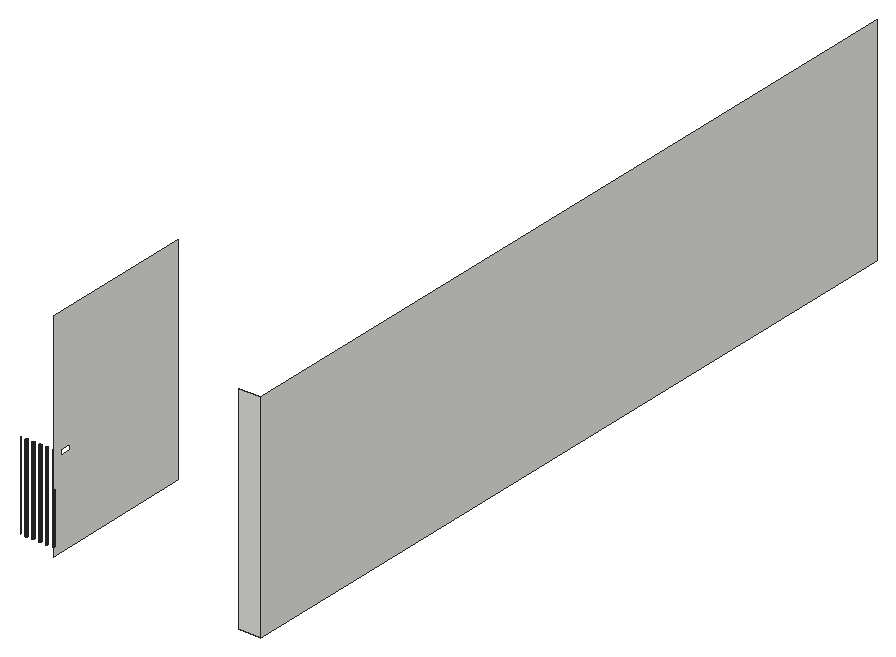
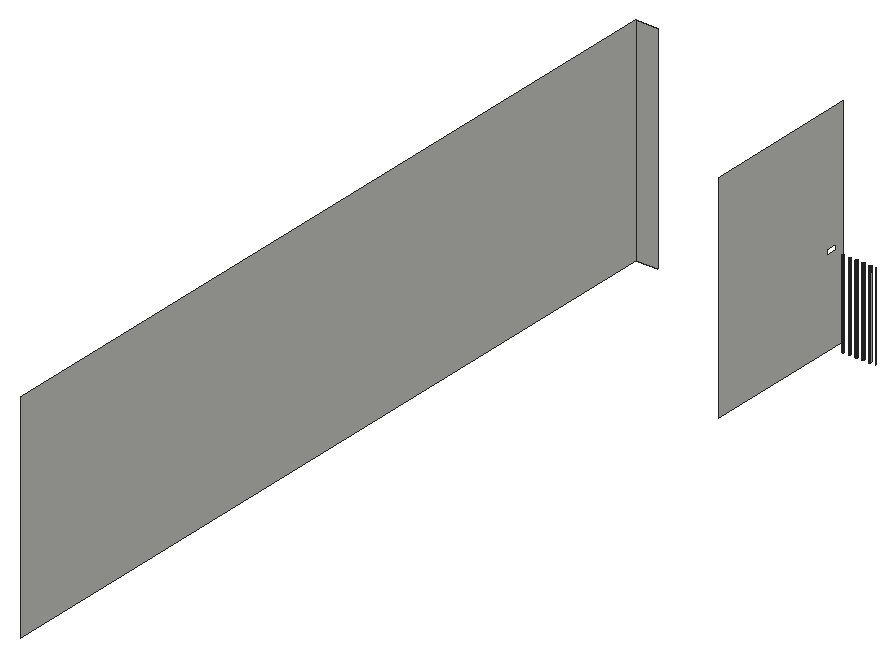
# SketchUp Ruby script. Lengths in inches.
U = 1.inch
M = Sketchup.active_model
def pt(a) = Geom::Point3d.new(a.map { |v| v * U })
def face(e, loops, mat)
  f = e.add_face(loops[0].map { |a| pt(a) })
  loops[1..].each { |l| e.add_face(l.map { |a| pt(a) }).erase! }
  f.material = f.back_material = mat if mat
  f
end
# faces: each face lists its corners as indices into pts; further lists are holes
def faces(e, pts, list, mat = nil) = list.each { |f| face(e, (f[0].is_a?(Array) ? f : [f]).map { |l| l.map { |i| pts[i] } }, mat) }
# xy, xz, yz: faces in a plane at the given z, y or x. An outline is a flat list of corners, or four numbers for a rectangle; further outlines are holes
def ring(l) = l.size == 4 ? [[l[0], l[1]], [l[2], l[1]], [l[2], l[3]], [l[0], l[3]]] : l.each_slice(2).to_a
def flat(e, list, mat, &to3) = list.each { |f| face(e, (f[0].is_a?(Array) ? f : [f]).map { |l| ring(l).map { |u, v| to3.(u, v) } }, mat) }
def xy(e, z, list, mat = nil) = flat(e, list, mat) { |x, y| [x, y, z] }
def xz(e, y, list, mat = nil) = flat(e, list, mat) { |x, z| [x, y, z] }
def yz(e, x, list, mat = nil) = flat(e, list, mat) { |y, z| [x, y, z] }
def lines(e, pts, list) = list.each { |a, b| e.add_line(pt(pts[a]), pt(pts[b])) }
# prism: a flat outline (further loops are holes) pulled along v
def prism(e, loops, v, mat = nil)
  f = face(e, loops, mat); d = Geom::Vector3d.new(v.map { |x| x * U })
  f.pushpull(f.normal.samedirection?(d) ? d.length : -d.length)
end
def box(e, o, s, mat = nil) = prism(e, [[o, [o[0] + s[0], o[1], o[2]], [o[0] + s[0], o[1] + s[1], o[2]], [o[0], o[1] + s[1], o[2]]]], [0, 0, s[2]], mat)
def at(x, y, z, deg = 0) = Geom::Transformation.translation(pt([x, y, z])) * Geom::Transformation.rotation(ORIGIN, Z_AXIS, deg.degrees)
def axes(o, x, y, z) = Geom::Transformation.new([*x, 0, *y, 0, *z, 0, *pt(o).to_a, 1])
def part(name) = M.definitions.add(name)
# library, detail: a bought-in or finely detailed component or shape, given as its bounding box
def library(name, o, s) = part(name).tap { |d| box(d.entities, o, s) }
def detail(e, o, s) = box(e.add_group.entities, o, s)
def put(e, d, t, mat = nil) = e.add_instance(d, t).tap { |i| i.material = mat if mat }
def group(e, t, mat = nil) = e.add_group.tap { |g| g.transformation = t; g.material = mat if mat }.entities
root = M.entities
xy(root,409.875,[[500.17,133.41,499.96,133.44,499.76,133.52,499.59,133.65,499.46,133.82,499.38,134.02,499.36,134.23,499.38,134.4375,499.46,134.63,499.59,134.8,499.76,134.93,499.96,135.01,500.17,135.04,500.38,135.01,500.57,134.93,500.74,134.8,500.87,134.63,500.95,134.4375,500.98,134.23,500.95,134.02,500.87,133.82,500.74,133.65,500.57,133.52,500.38,133.44],[505.42,133.41,505.21,133.44,505.01,133.52,504.84,133.65,504.71,133.82,504.63,134.02,504.61,134.23,504.63,134.4375,504.71,134.63,504.84,134.8,505.01,134.93,505.21,135.01,505.42,135.04,505.63,135.01,505.82,134.93,505.99,134.8,506.12,134.63,506.2,134.4375,506.23,134.23,506.2,134.02,506.12,133.82,505.99,133.65,505.82,133.52,505.63,133.44],[510.67,133.41,510.46,133.44,510.26,133.52,510.09,133.65,509.96,133.82,509.88,134.02,509.86,134.23,509.88,134.4375,509.96,134.63,510.09,134.8,510.26,134.93,510.46,135.01,510.67,135.04,510.88,135.01,511.07,134.93,511.24,134.8,511.37,134.63,511.45,134.4375,511.48,134.23,511.45,134.02,511.37,133.82,511.24,133.65,511.07,133.52,510.88,133.44],[515.92,133.41,515.71,133.44,515.51,133.52,515.34,133.65,515.21,133.82,515.13,134.02,515.11,134.23,515.13,134.4375,515.21,134.63,515.34,134.8,515.51,134.93,515.71,135.01,515.92,135.04,516.13,135.01,516.32,134.93,516.49,134.8,516.62,134.63,516.7,134.4375,516.73,134.23,516.7,134.02,516.62,133.82,516.49,133.65,516.32,133.52,516.13,133.44],[521.23,133.41,521.02,133.44,520.82,133.52,520.66,133.65,520.53,133.82,520.45,134.02,520.42,134.23,520.45,134.4375,520.53,134.63,520.66,134.8,520.82,134.93,521.02,135.01,521.23,135.04,521.44,135.01,521.64,134.93,521.8,134.8,521.93,134.63,522.02,134.4375,522.04,134.23,522.02,134.02,521.93,133.82,521.8,133.65,521.64,133.52,521.44,133.44]])
xz(root,124.5,[[673.48,409.875,690.4375,577.875]])
yz(root,528.75,[[[124.5,409.875,246,577.875],[131.37,477.08,140.67,481.27]]])
yz(root,690.4375,[[124.5,409.875,724.5,577.875]])
p = [[499.76,133.52,409.875],[499.96,133.44,409.875],[499.96,133.44,477.08],[499.76,133.52,477.08],[500.17,133.41,409.875],[500.17,133.41,477.08],
  [500.38,133.44,409.875],[500.38,133.44,477.08],[500.57,133.52,409.875],[500.57,133.52,477.08],[505.01,133.52,409.875],[505.21,133.44,409.875],
  [505.21,133.44,477.08],[505.01,133.52,477.08],[505.42,133.41,409.875],[505.42,133.41,477.08],[505.63,133.44,409.875],[505.63,133.44,477.08],
  [505.82,133.52,409.875],[505.82,133.52,477.08],[510.26,133.52,409.875],[510.46,133.44,409.875],[510.46,133.44,477.08],[510.26,133.52,477.08],
  [510.67,133.41,409.875],[510.67,133.41,477.08],[510.88,133.44,409.875],[510.88,133.44,477.08],[511.07,133.52,409.875],[511.07,133.52,477.08],
  [515.51,133.52,409.875],[515.71,133.44,409.875],[515.71,133.44,477.08],[515.51,133.52,477.08],[515.92,133.41,409.875],[515.92,133.41,477.08],
  [516.13,133.44,409.875],[516.13,133.44,477.08],[516.32,133.52,409.875],[516.32,133.52,477.08],[520.82,133.52,409.875],[521.02,133.44,409.875],
  [521.02,133.44,477.08],[520.82,133.52,477.08],[521.23,133.41,409.875],[521.23,133.41,477.08],[521.44,133.44,409.875],[521.44,133.44,477.08],
  [521.64,133.52,409.875],[521.64,133.52,477.08],[499.59,133.65,409.875],[499.59,133.65,477.08],[500.74,133.65,409.875],[500.74,133.65,477.08],
  [504.84,133.65,409.875],[504.84,133.65,477.08],[505.99,133.65,409.875],[505.99,133.65,477.08],[510.09,133.65,409.875],[510.09,133.65,477.08],
  [511.24,133.65,409.875],[511.24,133.65,477.08],[515.34,133.65,409.875],[515.34,133.65,477.08],[516.49,133.65,409.875],[516.49,133.65,477.08],
  [520.66,133.65,409.875],[520.66,133.65,477.08],[521.8,133.65,409.875],[521.8,133.65,477.08],[499.46,133.82,409.875],[499.46,133.82,477.08],
  [500.87,133.82,409.875],[500.87,133.82,477.08],[504.71,133.82,409.875],[504.71,133.82,477.08],[506.12,133.82,409.875],[506.12,133.82,477.08],
  [509.96,133.82,409.875],[509.96,133.82,477.08],[511.37,133.82,409.875],[511.37,133.82,477.08],[515.21,133.82,409.875],[515.21,133.82,477.08],
  [516.62,133.82,409.875],[516.62,133.82,477.08],[520.53,133.82,409.875],[520.53,133.82,477.08],[521.93,133.82,409.875],[521.93,133.82,477.08],
  [495.56,133.82,409.875],[495.64,134.02,409.875],[495.64,134.02,477.08],[495.56,133.82,477.08],[499.38,134.02,409.875],[499.38,134.02,477.08],
  [500.95,134.02,409.875],[500.95,134.02,477.08],[504.63,134.02,409.875],[504.63,134.02,477.08],[506.2,134.02,409.875],[506.2,134.02,477.08],
  [509.88,134.02,409.875],[509.88,134.02,477.08],[511.45,134.02,409.875],[511.45,134.02,477.08],[515.13,134.02,409.875],[515.13,134.02,477.08],
  [516.7,134.02,409.875],[516.7,134.02,477.08],[520.45,134.02,409.875],[520.45,134.02,477.08],[522.02,134.02,409.875],[522.02,134.02,477.08],
  [495.67,134.23,409.875],[495.67,134.23,477.08],[499.36,134.23,409.875],[499.36,134.23,477.08],[500.98,134.23,409.875],[500.98,134.23,477.08],
  [504.61,134.23,409.875],[504.61,134.23,477.08],[506.23,134.23,409.875],[506.23,134.23,477.08],[509.86,134.23,409.875],[509.86,134.23,477.08],
  [511.48,134.23,409.875],[511.48,134.23,477.08],[515.11,134.23,409.875],[515.11,134.23,477.08],[516.73,134.23,409.875],[516.73,134.23,477.08],
  [520.42,134.23,409.875],[520.42,134.23,477.08],[522.04,134.23,409.875],[522.04,134.23,477.08],[495.64,134.4375,409.875],[495.64,134.4375,477.08],
  [499.38,134.4375,409.875],[499.38,134.4375,477.08],[500.95,134.4375,409.875],[500.95,134.4375,477.08],[504.63,134.4375,409.875],[504.63,134.4375,477.08],
  [506.2,134.4375,409.875],[506.2,134.4375,477.08],[509.88,134.4375,409.875],[509.88,134.4375,477.08],[511.45,134.4375,409.875],[511.45,134.4375,477.08],
  [515.13,134.4375,409.875],[515.13,134.4375,477.08],[516.7,134.4375,409.875],[516.7,134.4375,477.08],[520.45,134.4375,409.875],[520.45,134.4375,477.08],
  [522.02,134.4375,409.875],[522.02,134.4375,477.08],[499.46,134.63,409.875],[499.46,134.63,477.08],[500.87,134.63,409.875],[500.87,134.63,477.08],
  [504.71,134.63,409.875],[504.71,134.63,477.08],[506.12,134.63,409.875],[506.12,134.63,477.08],[509.96,134.63,409.875],[509.96,134.63,477.08],
  [511.37,134.63,409.875],[511.37,134.63,477.08],[515.21,134.63,409.875],[515.21,134.63,477.08],[516.62,134.63,409.875],[516.62,134.63,477.08],
  [520.53,134.63,409.875],[520.53,134.63,477.08],[521.93,134.63,409.875],[521.93,134.63,477.08],[499.59,134.8,409.875],[499.59,134.8,477.08],
  [500.74,134.8,409.875],[500.74,134.8,477.08],[504.84,134.8,409.875],[504.84,134.8,477.08],[505.99,134.8,409.875],[505.99,134.8,477.08],
  [510.09,134.8,409.875],[510.09,134.8,477.08],[511.24,134.8,409.875],[511.24,134.8,477.08],[515.34,134.8,409.875],[515.34,134.8,477.08],
  [516.49,134.8,409.875],[516.49,134.8,477.08],[520.66,134.8,409.875],[520.66,134.8,477.08],[521.8,134.8,409.875],[521.8,134.8,477.08],
  [499.76,134.93,409.875],[499.76,134.93,477.08],[500.57,134.93,409.875],[500.57,134.93,477.08],[505.01,134.93,409.875],[505.01,134.93,477.08],
  [505.82,134.93,409.875],[505.82,134.93,477.08],[510.26,134.93,409.875],[510.26,134.93,477.08],[511.07,134.93,409.875],[511.07,134.93,477.08],
  [515.51,134.93,409.875],[515.51,134.93,477.08],[516.32,134.93,409.875],[516.32,134.93,477.08],[520.82,134.93,409.875],[520.82,134.93,477.08],
  [521.64,134.93,409.875],[521.64,134.93,477.08],[499.96,135.01,409.875],[499.96,135.01,477.08],[500.38,135.01,409.875],[500.38,135.01,477.08],
  [505.21,135.01,409.875],[505.21,135.01,477.08],[505.63,135.01,409.875],[505.63,135.01,477.08],[510.46,135.01,409.875],[510.46,135.01,477.08],
  [510.88,135.01,409.875],[510.88,135.01,477.08],[515.71,135.01,409.875],[515.71,135.01,477.08],[516.13,135.01,409.875],[516.13,135.01,477.08],
  [521.02,135.01,409.875],[521.02,135.01,477.08],[521.44,135.01,409.875],[521.44,135.01,477.08],[500.17,135.04,409.875],[500.17,135.04,477.08],
  [505.42,135.04,409.875],[505.42,135.04,477.08],[510.67,135.04,409.875],[510.67,135.04,477.08],[515.92,135.04,409.875],[515.92,135.04,477.08],
  [521.23,135.04,409.875],[521.23,135.04,477.08],[521.39,134.22,477.08],[521.39,134.22,409.875],[516.07,134.22,477.08],[516.07,134.22,409.875],
  [510.76,134.22,477.08],[510.76,134.22,409.875],[505.45,134.22,477.08],[505.45,134.22,409.875],[500.14,134.22,477.08],[500.14,134.22,409.875]]
faces(root,p,[[0,1,2,3],[1,4,5,2],[4,6,7,5],[6,8,9,7],[10,11,12,13],[11,14,15,12],[14,16,17,15],[16,18,19,17],
  [20,21,22,23],[21,24,25,22],[24,26,27,25],[26,28,29,27],[30,31,32,33],[31,34,35,32],[34,36,37,35],[36,38,39,37],
  [40,41,42,43],[41,44,45,42],[44,46,47,45],[46,48,49,47],[50,0,3,51],[8,52,53,9],[54,10,13,55],[18,56,57,19],
  [58,20,23,59],[28,60,61,29],[62,30,33,63],[38,64,65,39],[66,40,43,67],[48,68,69,49],[70,50,51,71],[52,72,73,53],
  [74,54,55,75],[56,76,77,57],[78,58,59,79],[60,80,81,61],[82,62,63,83],[64,84,85,65],[86,66,67,87],[68,88,89,69],
  [90,91,92,93],[94,70,71,95],[72,96,97,73],[98,74,75,99],[76,100,101,77],[102,78,79,103],[80,104,105,81],[106,82,83,107],
  [84,108,109,85],[110,86,87,111],[88,112,113,89],[91,114,115,92],[116,94,95,117],[96,118,119,97],[120,98,99,121],[100,122,123,101],
  [124,102,103,125],[104,126,127,105],[128,106,107,129],[108,130,131,109],[132,110,111,133],[112,134,135,113],[114,136,137,115],[138,116,117,139],
  [118,140,141,119],[142,120,121,143],[122,144,145,123],[146,124,125,147],[126,148,149,127],[150,128,129,151],[130,152,153,131],[154,132,133,155],
  [134,156,157,135],[158,138,139,159],[140,160,161,141],[162,142,143,163],[144,164,165,145],[166,146,147,167],[148,168,169,149],[170,150,151,171],
  [152,172,173,153],[174,154,155,175],[156,176,177,157],[178,158,159,179],[160,180,181,161],[182,162,163,183],[164,184,185,165],[186,166,167,187],
  [168,188,189,169],[190,170,171,191],[172,192,193,173],[194,174,175,195],[176,196,197,177],[198,178,179,199],[180,200,201,181],[202,182,183,203],
  [184,204,205,185],[206,186,187,207],[188,208,209,189],[210,190,191,211],[192,212,213,193],[214,194,195,215],[196,216,217,197],[218,198,199,219],
  [200,220,221,201],[222,202,203,223],[204,224,225,205],[226,206,207,227],[208,228,229,209],[230,210,211,231],[212,232,233,213],[234,214,215,235],
  [216,236,237,217],[238,218,219,239],[220,238,239,221],[240,222,223,241],[224,240,241,225],[242,226,227,243],[228,242,243,229],[244,230,231,245],
  [232,244,245,233],[246,234,235,247],[236,246,247,237]])
lines(root,p,[[248,249],[250,251],[252,253],[254,255],[256,257]])
